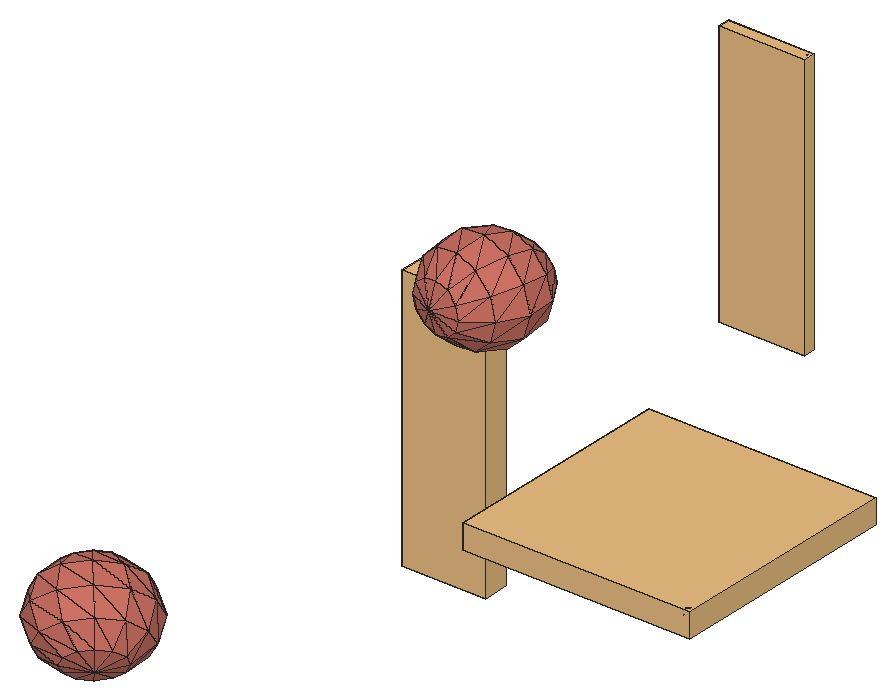
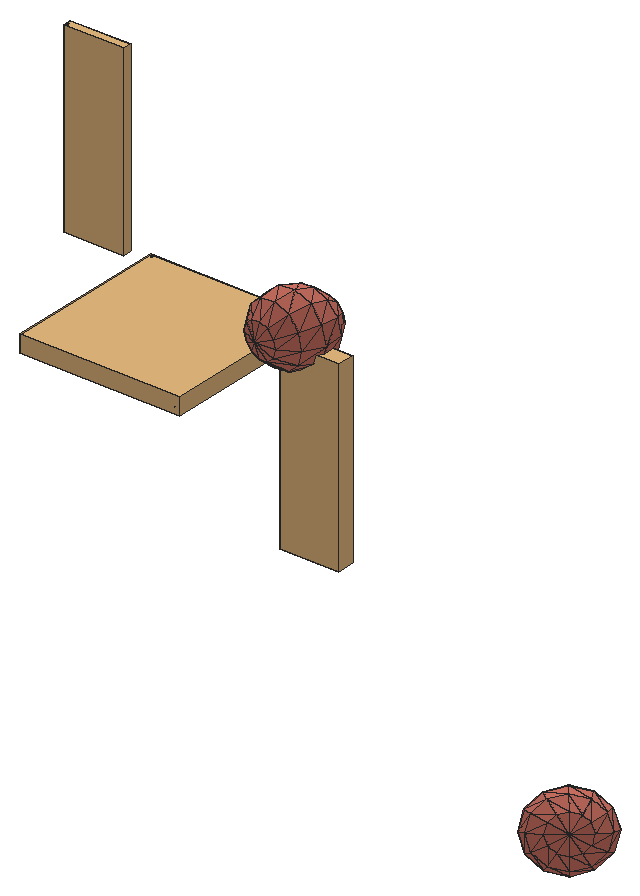
# SketchUp Ruby script. Lengths in inches.
U = 1.inch
M = Sketchup.active_model
def pt(a) = Geom::Point3d.new(a.map { |v| v * U })
def face(e, loops, mat)
  f = e.add_face(loops[0].map { |a| pt(a) })
  loops[1..].each { |l| e.add_face(l.map { |a| pt(a) }).erase! }
  f.material = f.back_material = mat if mat
  f
end
# faces: each face lists its corners as indices into pts; further lists are holes
def faces(e, pts, list, mat = nil) = list.each { |f| face(e, (f[0].is_a?(Array) ? f : [f]).map { |l| l.map { |i| pts[i] } }, mat) }
# xy, xz, yz: faces in a plane at the given z, y or x. An outline is a flat list of corners, or four numbers for a rectangle; further outlines are holes
def ring(l) = l.size == 4 ? [[l[0], l[1]], [l[2], l[1]], [l[2], l[3]], [l[0], l[3]]] : l.each_slice(2).to_a
def flat(e, list, mat, &to3) = list.each { |f| face(e, (f[0].is_a?(Array) ? f : [f]).map { |l| ring(l).map { |u, v| to3.(u, v) } }, mat) }
def xy(e, z, list, mat = nil) = flat(e, list, mat) { |x, y| [x, y, z] }
def xz(e, y, list, mat = nil) = flat(e, list, mat) { |x, z| [x, y, z] }
def yz(e, x, list, mat = nil) = flat(e, list, mat) { |y, z| [x, y, z] }
def lines(e, pts, list) = list.each { |a, b| e.add_line(pt(pts[a]), pt(pts[b])) }
# prism: a flat outline (further loops are holes) pulled along v
def prism(e, loops, v, mat = nil)
  f = face(e, loops, mat); d = Geom::Vector3d.new(v.map { |x| x * U })
  f.pushpull(f.normal.samedirection?(d) ? d.length : -d.length)
end
def box(e, o, s, mat = nil) = prism(e, [[o, [o[0] + s[0], o[1], o[2]], [o[0] + s[0], o[1] + s[1], o[2]], [o[0], o[1] + s[1], o[2]]]], [0, 0, s[2]], mat)
def at(x, y, z, deg = 0) = Geom::Transformation.translation(pt([x, y, z])) * Geom::Transformation.rotation(ORIGIN, Z_AXIS, deg.degrees)
def axes(o, x, y, z) = Geom::Transformation.new([*x, 0, *y, 0, *z, 0, *pt(o).to_a, 1])
def part(name) = M.definitions.add(name)
# library, detail: a bought-in or finely detailed component or shape, given as its bounding box
def library(name, o, s) = part(name).tap { |d| box(d.entities, o, s) }
def detail(e, o, s) = box(e.add_group.entities, o, s)
def put(e, d, t, mat = nil) = e.add_instance(d, t).tap { |i| i.material = mat if mat }
def group(e, t, mat = nil) = e.add_group.tap { |g| g.transformation = t; g.material = mat if mat }.entities
root = M.entities
M.materials.add("green").color = [174, 139, 102]
M.materials.add("vio").color = [206, 114, 100]
c1 = part("3DGeom~202_Defintion")
p = [[2.15,-326.37,-327.67],[-168.31,-180.33,-426.3],[-6.92,-60.875,-500],[2.15,-326.37,-327.67],[188.51,-188.43,-412.77],[188.51,-188.43,-412.77],
  [110.74,102.31,-477.91],[-200.49,82.99,-453.25],[-132.5625,177.21,-440.5],[188.51,-188.43,-412.77],[324.36,0,-387.27],[324.36,0,-387.27],
  [153.12,265.49,-365.96],[-108.09,271.42,-375.87],[-108.09,271.42,-375.87],[153.12,265.49,-365.96],[-293.67,14.02,-410.7],[-340.34,204.62,-285.05],
  [-340.34,204.62,-285.05],[-108.09,271.42,-375.87],[-340.34,204.62,-285.05],[-184.79,-376.86,-154.77],[-330.2,-224.0625,-276.5625],[-184.79,-376.86,-154.77],
  [2.15,-326.37,-327.67],[-330.2,-224.0625,-276.5625],[172.03,-384.95,-141.25],[2.15,-326.37,-327.67],[188.51,-188.43,-412.77],[188.51,-188.43,-412.77],
  [333.43,-265.49,-214.95],[333.43,-265.49,-214.95],[188.51,-188.43,-412.77],[324.36,0,-387.27],[-330.2,-224.0625,-276.5625],[-387.14,-11.23,-324.25],
  [-293.67,14.02,-410.7],[-387.14,-11.23,-324.25],[-340.34,204.62,-285.05],[451.08,-102.31,-192.86],[373.3,188.43,-258],[324.36,0,-387.27],
  [153.12,265.49,-365.96],[373.3,188.43,-258],[-133.64,340.39,-276.66],[-108.09,271.42,-375.87],[-340.34,204.62,-285.05],[153.12,265.49,-365.96],
  [-108.09,271.42,-375.87],[-133.64,340.39,-276.66],[373.3,188.43,-258],[108.875,384.95,-194.14],[10.14,-428.68,8.49],[-184.79,-376.86,-154.77],
  [-449.22,-180.33,-90.91],[-330.2,-224.0625,-276.5625],[-455.85,14.02,-217.06],[-481.39,82.99,-117.86],[-456.93,177.2,-53.23],[-389,271.42,-40.48],
  [-295.82,340.39,-83.03],[-295.82,340.39,-83.03],[-202.35,365.63,-169.48],[-202.35,365.63,-169.48],[-340.34,204.62,-285.05],[-322.21,-326.37,59.6],
  [-184.79,-376.86,-154.77],[-322.21,-326.37,59.6],[493.46,60.875,-80.91],[322.21,326.37,-59.6],[373.3,188.43,-258],[322.21,326.37,-59.6],
  [-493.46,-60.875,80.91],[295.82,-340.39,83.03],[333.43,-265.49,-214.95],[295.82,-340.39,83.03],[333.43,-265.49,-214.95],[389,-271.42,40.48],
  [389,-271.42,40.48],[322.21,326.37,-59.6],[-10.14,428.68,-8.49],[456.93,-177.2,53.23],[-295.82,340.39,-83.03],[-108.875,-384.95,194.14],
  [-322.21,-326.37,59.6],[202.35,-365.63,169.48],[295.82,-340.39,83.03],[-451.08,102.31,192.86],[-373.3,-188.43,258],[-322.21,-326.37,59.6],
  [-373.3,-188.43,258],[-172.03,384.95,141.25],[-389,271.42,-40.48],[481.39,-82.99,117.86],[449.22,180.33,90.91],[184.79,376.86,154.77],
  [322.21,326.37,-59.6],[184.79,376.86,154.77],[-333.43,265.49,214.95],[-389,271.42,-40.48],[-333.43,265.49,214.95],[184.79,376.86,154.77],
  [133.64,-340.39,276.66],[295.82,-340.39,83.03],[340.34,-204.62,285.05],[340.34,-204.62,285.05],[340.34,-204.62,285.05],[-153.12,-265.49,365.96],
  [-373.3,-188.43,258],[-324.36,0,387.27],[-373.3,-188.43,258],[-324.36,0,387.27],[202.35,-365.63,169.48],[340.34,-204.62,285.05],
  [455.85,-14.02,217.07],[330.2,224.0625,276.5625],[184.79,376.86,154.77],[330.2,224.0625,276.5625],[340.34,-204.62,285.05],[-2.15,326.37,327.67],
  [-333.43,265.49,214.95],[184.79,376.86,154.77],[-2.15,326.37,327.67],[330.2,224.0625,276.5625],[184.79,376.86,154.77],[-2.15,326.37,327.67],
  [340.34,-204.62,285.05],[-188.51,188.43,412.77],[-324.36,0,387.27],[-188.51,188.43,412.77],[108.09,-271.42,375.87],[108.09,-271.42,375.87],
  [-2.15,326.37,327.67],[-333.43,265.49,214.95],[-188.51,188.43,412.77],[387.14,11.23,324.25],[340.34,-204.62,285.05],[330.2,224.0625,276.5625],
  [-110.74,-102.31,477.91],[-373.3,-188.43,258],[-153.12,-265.49,365.96],[-324.36,0,387.27],[-373.3,-188.43,258],[387.14,11.23,324.25],
  [168.31,180.33,426.3],[108.09,-271.42,375.87],[133.64,-340.39,276.66],[340.34,-204.62,285.05],[132.5625,-177.21,440.5],[340.34,-204.62,285.05],
  [200.49,-82.99,453.25],[340.34,-204.62,285.05],[293.67,-14.02,410.7],[340.34,-204.62,285.05],[293.67,-14.02,410.7],[340.34,-204.62,285.05],
  [387.14,11.23,324.25],[-188.51,188.43,412.77],[-153.12,-265.49,365.96],[-153.12,-265.49,365.96],[6.92,60.875,500]]
faces(c1.entities,p,[[0,1,2],[3,2,4],[5,2,6],[1,7,2],[2,7,8],[2,8,6],[9,6,10],[11,6,12],
  [6,8,13],[6,14,15],[1,16,7],[7,16,17],[8,7,18],[19,8,20],[21,22,1],[23,1,24],
  [25,16,1],[26,27,28],[26,29,30],[31,32,33],[34,35,16],[36,37,38],[31,33,39],[39,33,40],
  [41,42,43],[44,45,46],[47,48,49],[50,47,51],[47,49,51],[52,53,27],[52,27,26],[54,37,55],
  [54,56,37],[37,56,38],[56,57,38],[57,58,38],[58,59,38],[59,60,38],[61,62,38],[63,49,64],
  [51,49,63],[65,55,66],[67,54,55],[39,40,68],[68,40,69],[70,51,71],[72,56,54],[72,57,56],
  [73,26,74],[75,76,77],[78,31,39],[79,51,80],[51,63,80],[78,39,81],[81,39,68],[80,63,82],
  [83,53,52],[83,84,53],[85,52,26],[85,26,86],[87,57,72],[87,58,57],[88,54,89],[90,72,54],
  [91,82,92],[80,82,91],[81,68,93],[93,68,94],[68,69,94],[94,69,95],[96,80,97],[98,58,87],
  [98,59,58],[91,99,100],[101,80,91],[102,83,52],[102,52,85],[103,78,104],[78,81,105],[81,93,106],
  [107,84,83],[107,108,84],[109,72,110],[111,87,72],[112,103,113],[93,94,114],[114,94,115],[94,116,117],
  [93,114,118],[119,91,120],[121,91,122],[123,124,125],[102,85,126],[127,87,128],[129,98,87],[130,107,83],
  [131,83,102],[132,133,134],[114,135,136],[114,137,135],[138,139,140],[138,141,142],[143,123,144],[123,125,144],
  [145,146,147],[148,145,149],[150,148,151],[152,150,153],[135,154,155],[156,144,152],[144,125,157],[148,158,145],
  [148,138,159],[160,141,138],[160,157,141],[152,160,150],[152,144,160],[144,157,160],[150,138,148],[150,160,138]],"vio")
c2 = library("3DGeom~123_Defintion",[-47.43,-500,-158.67],[94.86,1000,317.34])
c3 = part("3DGeom~124_Defintion")
p = [[-44.78,-498.52,-137.32],[-32.6875,-500,-148.14],[-41.35,-495.57,-121.75],[-32.6875,-500,-148.14],[-44.78,-498.52,-137.32],[-40.2,-499.6,-144.3],
  [-41.35,-495.57,-121.75],[-32.6875,-500,-148.14],[-25.84,-494.09,-117],[-32.6875,-500,-148.14],[-24.26,-499.6,-147.81],[-17.18,-498.52,-143.39],
  [-13.75,-495.57,-127.82],[-32.6875,-500,-148.14],[-17.18,-498.52,-143.39],[-25.84,-494.09,-117],[-32.6875,-500,-148.14],[-13.75,-495.57,-127.82],
  [-13.75,-495.57,-127.82],[-17.18,-498.52,-143.39],[-13.33,-497.04,-136.08],[-44.78,-498.52,-137.32],[-41.35,-495.57,-121.75],[-45.2,-497.04,-129.06],
  [-25.84,-494.09,-117],[-13.75,-495.57,-127.82],[-18.33,-494.49,-120.84],[-41.35,-495.57,-121.75],[-25.84,-494.09,-117],[-34.27,-494.49,-117.33],
  [28.19,500,128.65],[26.39,491.3,158.41],[34.8,490.68,158.67],[28.19,500,128.65],[34.8,490.68,158.67],[42.32,491.3,154.91],
  [28.19,500,128.65],[19.34,493.01,154.2],[26.39,491.3,158.41],[28.19,500,128.65],[42.32,491.3,154.91],[46.95,493.01,148.13],
  [28.19,500,128.65],[15.56,495.34,147.17],[19.34,493.01,154.2],[28.19,500,128.65],[46.95,493.01,148.13],[47.43,495.34,140.16],
  [28.19,500,128.65],[16.04,497.67,139.19],[15.56,495.34,147.17],[28.19,500,128.65],[47.43,495.34,140.16],[43.65,497.67,133.12],
  [28.19,500,128.65],[20.67,499.375,132.42],[16.04,497.67,139.19],[28.19,500,128.65],[43.65,497.67,133.12],[36.61,499.375,128.91]]
faces(c3.entities,p,[[0,1,2],[3,4,5],[6,7,8],[9,10,11],[12,13,14],[15,16,17],[18,19,20],[21,22,23],
  [24,25,26],[27,28,29],[30,31,32],[33,34,35],[36,37,38],[39,40,41],[42,43,44],[45,46,47],
  [48,49,50],[51,52,53],[54,55,56],[57,58,59]],"green")
c4 = part("3DGeom~228_Defintion")
p = [[-95.24,-217.29,-433.01],[-345.24,0,-378.02],[-109.98,0,-500],[167.52,-188.18,-429.99],[154.76,0,-488],[-332.48,188.18,-320.01],
  [-95.24,217.29,-433.01],[385.39,-108.65,-311.75],[385.39,-108.65,-311.75],[378.02,0,-345.24],[167.52,188.18,-429.99],[378.02,0,-345.24],
  [-54.99,-376.36,-250],[-332.48,-188.18,-320.01],[202.38,-325.94,-271.5],[-297.62,325.94,-161.52],[-54.99,376.36,-250],[-297.62,325.94,-161.52],
  [-54.99,376.36,-250],[405.52,-188.18,-220.24],[405.52,-188.18,-220.24],[385.39,-108.65,-311.75],[378.02,0,-345.24],[385.39,108.65,-311.75],
  [385.39,108.65,-311.75],[202.38,325.94,-271.5],[-54.99,376.36,-250],[202.38,325.94,-271.5],[-332.48,-188.18,-320.01],[-488,0,-154.76],
  [-345.24,0,-378.02],[-345.24,0,-378.02],[-480.63,108.65,-121.26],[-345.24,0,-378.02],[-332.48,188.18,-320.01],[385.39,-108.65,-311.75],
  [378.02,0,-345.24],[500,0,-109.98],[385.39,108.65,-311.75],[-297.62,-325.94,-161.52],[-297.62,-325.94,-161.52],[-480.63,-108.65,-121.26],
  [-332.48,-188.18,-320.01],[-332.48,-188.18,-320.01],[-332.48,188.18,-320.01],[-460.51,188.18,-29.76],[-332.48,188.18,-320.01],[-297.62,325.94,-161.52],
  [405.52,-188.18,-220.24],[405.52,188.18,-220.24],[385.39,108.65,-311.75],[202.38,325.94,-271.5],[405.52,188.18,-220.24],[250,-376.36,-54.99],
  [-54.99,-376.36,-250],[202.38,-325.94,-271.5],[433.01,-217.29,-95.24],[250,-376.36,-54.99],[202.38,-325.94,-271.5],[202.38,-325.94,-271.5],
  [202.38,325.94,-271.5],[250,376.36,-54.99],[202.38,325.94,-271.5],[-54.99,376.36,-250],[0,434.59,0],[202.38,325.94,-271.5],
  [250,376.36,-54.99],[0,-434.59,0],[-297.62,-325.94,-161.52],[-54.99,-376.36,-250],[250,-376.36,-54.99],[-54.99,-376.36,-250],
  [-297.62,325.94,-161.52],[-250,376.36,54.99],[433.01,217.29,-95.24],[-250,-376.36,54.99],[-297.62,-325.94,-161.52],[-250,-376.36,54.99],
  [-460.51,-188.18,-29.76],[-297.62,-325.94,-161.52],[-297.62,-325.94,-161.52],[-297.62,325.94,-161.52],[-433.01,217.29,95.24],[-297.62,325.94,-161.52],
  [-250,376.36,54.99],[-500,0,109.98],[460.51,-188.18,29.76],[480.64,-108.65,121.26],[488,0,154.76],[460.51,188.18,29.76],
  [480.64,108.65,121.26],[297.625,325.94,161.52],[297.62,-325.94,161.52],[250,-376.36,-54.99],[297.62,-325.94,161.52],[250,376.36,-54.99],
  [54.99,376.36,250],[297.625,325.94,161.52],[250,376.36,-54.99],[54.99,376.36,250],[-250,-376.36,54.99],[-433.01,-217.29,95.24],
  [54.99,-376.36,250],[297.62,-325.94,161.52],[-202.375,325.94,271.5],[-202.375,325.94,271.5],[54.99,376.36,250],[332.49,188.18,320.01],
  [-202.38,-325.94,271.5],[-250,-376.36,54.99],[-202.38,-325.94,271.5],[-250,376.36,54.99],[-405.52,188.18,220.24],[-250,376.36,54.99],
  [-405.52,188.18,220.24],[-202.375,325.94,271.5],[-202.38,-325.94,271.5],[-405.52,-188.18,220.24],[-405.52,188.18,220.24],[-385.39,-108.65,311.75],
  [-385.39,-108.65,311.75],[-378.02,0,345.24],[-378.02,0,345.24],[-385.39,108.65,311.75],[-385.39,108.65,311.75],[-405.52,188.18,220.24],
  [332.48,-188.18,320.01],[345.24,0,378.02],[332.48,-188.18,320.01],[54.99,-376.36,250],[297.62,-325.94,161.52],[297.625,325.94,161.52],
  [95.25,217.29,433.01],[332.49,188.18,320.01],[297.625,325.94,161.52],[54.99,376.36,250],[-167.52,-188.18,429.99],[-405.52,-188.18,220.24],
  [-202.38,-325.94,271.5],[-385.39,-108.65,311.75],[-405.52,-188.18,220.24],[-202.375,325.94,271.5],[-405.52,188.18,220.24],[-385.39,108.65,311.75],
  [95.24,-217.29,433.01],[-202.38,-325.94,271.5],[54.99,-376.36,250],[332.48,-188.18,320.01],[54.99,-376.36,250],[-167.51,188.18,429.99],
  [-202.38,-325.94,271.5],[-154.76,0,488],[-378.02,0,345.24],[345.24,0,378.02],[332.48,-188.18,320.01],[332.49,188.18,320.01],
  [109.98,0,500],[332.49,188.18,320.01],[345.24,0,378.02],[345.24,0,378.02]]
faces(c4.entities,p,[[0,1,2],[3,0,2],[3,2,4],[2,1,5],[2,5,6],[4,2,6],[7,3,4],[8,4,9],
  [4,6,10],[11,4,10],[12,13,0],[14,12,0],[14,0,3],[0,13,1],[6,5,15],[10,6,16],
  [6,17,18],[19,14,3],[20,3,21],[22,10,23],[24,10,25],[10,26,27],[28,29,30],[31,29,32],
  [33,32,34],[35,36,37],[36,38,37],[12,39,13],[40,41,42],[43,41,29],[44,32,45],[46,45,47],
  [48,35,37],[38,49,37],[50,51,52],[53,54,55],[56,57,58],[56,59,48],[49,60,61],[62,63,64],
  [65,64,66],[67,68,69],[70,67,71],[63,72,73],[63,73,64],[56,48,37],[49,74,37],[49,61,74],
  [67,75,76],[77,78,79],[80,78,41],[81,45,82],[83,82,84],[29,41,85],[32,29,85],[41,78,85],
  [45,32,85],[86,56,37],[87,86,37],[88,87,37],[74,89,37],[89,90,37],[90,88,37],[86,57,56],
  [74,91,89],[74,61,91],[92,67,93],[86,94,57],[95,96,97],[98,64,99],[100,101,78],[78,101,85],
  [82,45,85],[102,75,67],[103,102,67],[64,73,104],[64,105,106],[87,94,86],[89,107,90],[89,91,107],
  [108,101,109],[102,110,75],[111,82,112],[113,114,115],[116,117,101],[101,117,85],[118,82,85],[117,119,85],
  [120,121,85],[122,123,85],[124,125,85],[87,126,94],[88,126,87],[90,107,127],[90,127,88],[88,127,126],
  [128,129,130],[131,132,133],[134,135,132],[136,137,138],[136,139,140],[141,142,143],[144,145,146],[147,144,148],
  [135,141,149],[135,149,132],[144,136,150],[141,143,149],[151,139,136],[151,152,139],[149,143,152],[153,144,154],
  [155,132,156],[157,156,158],[149,152,151],[159,156,144],[156,136,144],[156,151,136],[132,149,151],[132,151,156]],"vio")
c5 = library("3DGeom~125_Defintion",[-500,-52.11,-487.65],[1000,104.22,975.3])
c6 = part("3DGeom~126_Defintion")
p = [[-471.41,-45.23,-481.51],[-492.01,-24.59,-479.28],[-477.71,-31.47,-487.65],[-471.41,-45.23,-481.51],[-477.71,-31.47,-487.65],[-472.84,-38.35,-486.35],
  [-492.01,-24.59,-479.28],[-484.73,-26.43,-485.0625],[-477.71,-31.47,-487.65],[-479.4,-52.11,-467],[-492.01,-24.59,-479.28],[-471.41,-45.23,-481.51],
  [-479.4,-52.11,-467],[-471.41,-45.23,-481.51],[-473.8125,-50.26,-474.43],[-493.7,-45.23,-458.63],[-492.01,-24.59,-479.28],[-479.4,-52.11,-467],
  [-500,-31.47,-464.77],[-492.01,-24.59,-479.28],[-493.7,-45.23,-458.63],[-492.01,-24.59,-479.28],[-497.6,-26.43,-471.85],[-493.7,-45.23,-458.63],
  [-479.4,-52.11,-467],[-486.68,-50.26,-461.22],[-493.7,-45.23,-458.63],[-498.57,-38.35,-459.93],[487.9375,29.11,475.22],[497.875,5.67,462.61],
  [500,13.48,461.23],[487.9375,29.11,475.22],[498.68,21.29,463.39],[487.9375,29.11,475.22],[492.87,-0.05,467.15],[497.875,5.67,462.61],
  [487.9375,29.11,475.22],[498.68,21.29,463.39],[494.26,27.01,468.51],[487.9375,29.11,475.22],[486.33,-2.15,473.66],[492.87,-0.05,467.15],
  [487.9375,29.11,475.22],[480,-0.05,480.37],[486.33,-2.15,473.66],[487.9375,29.11,475.22],[475.59,5.67,485.49],[480,-0.05,480.37],
  [487.9375,29.11,475.22],[474.26,13.48,487.65],[475.59,5.67,485.49],[487.9375,29.11,475.22],[476.39,21.29,486.27],[474.26,13.48,487.65],
  [487.9375,29.11,475.22],[481.39,27.01,481.72],[476.39,21.29,486.27]]
faces(c6.entities,p,[[0,1,2],[3,4,5],[6,7,8],[9,10,11],[12,13,14],[15,16,17],[18,19,20],[21,18,22],
  [23,24,25],[18,26,27],[28,29,30],[31,30,32],[33,34,35],[36,37,38],[39,40,41],[42,43,44],
  [45,46,47],[48,49,50],[51,52,53],[54,55,56]],"green")
c7 = library("3DGeom~119_Defintion",[-23.33,-500,-162.27],[46.66,1000,324.54])
c8 = part("3DGeom~120_Defintion")
p = [[-7.96,-495.57,-128.3],[7.3,-500,-151.51],[5.77,-494.09,-119.66],[-7.2,-498.52,-144.22],[7.3,-500,-151.51],[-7.96,-495.57,-128.3],
  [7.3,-500,-151.51],[-7.2,-498.52,-144.22],[-0.95,-499.6,-149.76],[5.77,-494.09,-119.66],[7.3,-500,-151.51],[20.27,-495.57,-126.94],
  [7.3,-500,-151.51],[15.35,-499.6,-148.98],[21.03,-498.52,-142.87],[20.27,-495.57,-126.94],[7.3,-500,-151.51],[21.03,-498.52,-142.87],
  [-7.2,-498.52,-144.22],[-7.96,-495.57,-128.3],[-9.76,-497.04,-136.37],[20.27,-495.57,-126.94],[21.03,-498.52,-142.87],[22.83,-497.04,-134.8],
  [-7.96,-495.57,-128.3],[5.77,-494.09,-119.66],[-2.28,-494.49,-122.18],[5.77,-494.09,-119.66],[20.27,-495.57,-126.94],[14.02,-494.49,-121.4],
  [-6.3,500,131.58],[-15.82,491.3,159.83],[-7.77,490.68,162.27],[-6.3,500,131.58],[-7.77,490.68,162.27],[0.48,491.3,160.61],
  [-6.3,500,131.58],[-21.52,493.01,153.92],[-15.82,491.3,159.83],[-6.3,500,131.58],[0.48,491.3,160.61],[6.71,493.01,155.28],
  [-6.3,500,131.58],[-23.33,495.34,146.14],[-21.52,493.01,153.92],[-6.3,500,131.58],[6.71,493.01,155.28],[9.26,495.34,147.71],
  [-6.3,500,131.58],[-20.78,497.67,138.57],[-23.33,495.34,146.14],[-6.3,500,131.58],[9.26,495.34,147.71],[7.45,497.67,139.93],
  [-6.3,500,131.58],[-14.55,499.375,133.24],[-20.78,497.67,138.57],[-6.3,500,131.58],[7.45,497.67,139.93],[1.75,499.375,134.03]]
faces(c8.entities,p,[[0,1,2],[3,4,5],[6,7,8],[9,10,11],[12,13,14],[15,16,17],[18,19,20],[21,22,23],
  [24,25,26],[27,28,29],[30,31,32],[33,34,35],[36,37,38],[39,40,41],[42,43,44],[45,46,47],
  [48,49,50],[51,52,53],[54,55,56],[57,58,59]],"green")
g1 = group(root,at(15.3125,38.42,26.21))
put(g1,c1,axes([-0.23,0.63,9.71],[0,0.00039,0],[0,0,-0.00039],[-0.00039,0,0]),"vio")
g2 = group(root,at(15.3125,38.42,26.21))
put(g2,c2,axes([1.13,0.48,10.83],[0,0.00091,0],[0,0,-0.00091],[-0.00091,0,0]),"green")
put(g2,c3,axes([1.13,0.48,10.83],[0,0.00091,0],[0,0,-0.00091],[-0.00091,0,0]),"green")
g3 = group(root,at(15.3125,38.42,26.21))
put(g3,c4,axes([1.26,0.45,11.32],[0,0.00038,0],[0,0,-0.00038],[-0.00038,0,0]),"vio")
g4 = group(root,at(15.3125,38.42,26.21))
put(g4,c5,axes([2.03,0.28,10.94],[0,0.0008,0],[0,0,-0.0008],[-0.0008,0,0]),"green")
put(g4,c6,axes([2.03,0.28,10.94],[0,0.0008,0],[0,0,-0.0008],[-0.0008,0,0]),"green")
g5 = group(root,at(15.3125,38.42,26.21))
put(g5,c7,axes([2.14,0.56,11.89],[0,0.00091,0],[0,0,-0.00091],[-0.00091,0,0]),"green")
put(g5,c8,axes([2.14,0.56,11.89],[0,0.00091,0],[0,0,-0.00091],[-0.00091,0,0]),"green")
